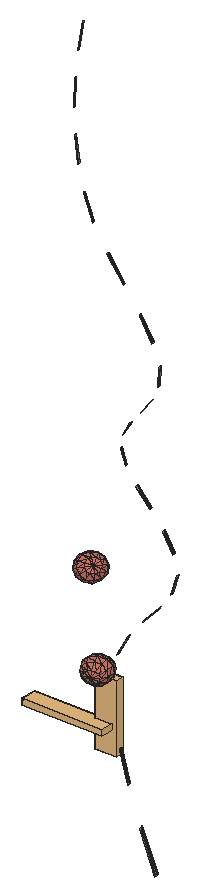
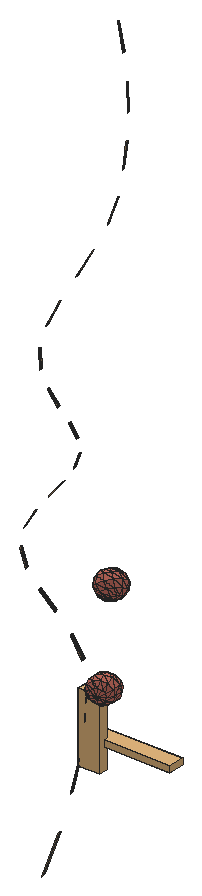
# SketchUp Ruby script. Lengths in inches.
U = 1.inch
M = Sketchup.active_model
def pt(a) = Geom::Point3d.new(a.map { |v| v * U })
def face(e, loops, mat)
  f = e.add_face(loops[0].map { |a| pt(a) })
  loops[1..].each { |l| e.add_face(l.map { |a| pt(a) }).erase! }
  f.material = f.back_material = mat if mat
  f
end
# faces: each face lists its corners as indices into pts; further lists are holes
def faces(e, pts, list, mat = nil) = list.each { |f| face(e, (f[0].is_a?(Array) ? f : [f]).map { |l| l.map { |i| pts[i] } }, mat) }
# xy, xz, yz: faces in a plane at the given z, y or x. An outline is a flat list of corners, or four numbers for a rectangle; further outlines are holes
def ring(l) = l.size == 4 ? [[l[0], l[1]], [l[2], l[1]], [l[2], l[3]], [l[0], l[3]]] : l.each_slice(2).to_a
def flat(e, list, mat, &to3) = list.each { |f| face(e, (f[0].is_a?(Array) ? f : [f]).map { |l| ring(l).map { |u, v| to3.(u, v) } }, mat) }
def xy(e, z, list, mat = nil) = flat(e, list, mat) { |x, y| [x, y, z] }
def xz(e, y, list, mat = nil) = flat(e, list, mat) { |x, z| [x, y, z] }
def yz(e, x, list, mat = nil) = flat(e, list, mat) { |y, z| [x, y, z] }
def lines(e, pts, list) = list.each { |a, b| e.add_line(pt(pts[a]), pt(pts[b])) }
# prism: a flat outline (further loops are holes) pulled along v
def prism(e, loops, v, mat = nil)
  f = face(e, loops, mat); d = Geom::Vector3d.new(v.map { |x| x * U })
  f.pushpull(f.normal.samedirection?(d) ? d.length : -d.length)
end
def box(e, o, s, mat = nil) = prism(e, [[o, [o[0] + s[0], o[1], o[2]], [o[0] + s[0], o[1] + s[1], o[2]], [o[0], o[1] + s[1], o[2]]]], [0, 0, s[2]], mat)
def at(x, y, z, deg = 0) = Geom::Transformation.translation(pt([x, y, z])) * Geom::Transformation.rotation(ORIGIN, Z_AXIS, deg.degrees)
def axes(o, x, y, z) = Geom::Transformation.new([*x, 0, *y, 0, *z, 0, *pt(o).to_a, 1])
def part(name) = M.definitions.add(name)
# library, detail: a bought-in or finely detailed component or shape, given as its bounding box
def library(name, o, s) = part(name).tap { |d| box(d.entities, o, s) }
def detail(e, o, s) = box(e.add_group.entities, o, s)
def put(e, d, t, mat = nil) = e.add_instance(d, t).tap { |i| i.material = mat if mat }
def group(e, t, mat = nil) = e.add_group.tap { |g| g.transformation = t; g.material = mat if mat }.entities
root = M.entities
M.materials.add("green").color = [174, 139, 102]
M.materials.add("vio").color = [206, 114, 100]
c1 = library("3DGeom~98_Defintion",[-97.72,-35.49,-500],[195.44,70.98,1000])
c2 = part("3DGeom~99_Defintion")
p = [[97.72,22.79,-497.94],[82.82,12.47,-499.74],[76.21,14.6,-500],[97.72,22.79,-497.94],[76.21,14.6,-500],[71.74,19.25,-499.92],
  [97.72,22.79,-497.94],[71.74,19.25,-499.92],[70.59,25.16,-499.53],[97.72,22.79,-497.94],[89.78,13.42,-499.21],[82.82,12.47,-499.74],
  [97.72,22.79,-497.94],[70.59,25.16,-499.53],[73.07,30.76,-498.92],[97.72,22.79,-497.94],[95.24,17.19,-498.55],[89.78,13.42,-499.21],
  [97.72,22.79,-497.94],[73.07,30.76,-498.92],[78.53,34.54,-498.26],[97.72,22.79,-497.94],[78.53,34.54,-498.26],[85.49,35.49,-497.73],
  [97.72,22.79,-497.94],[85.49,35.49,-497.73],[92.1,33.35,-497.47],[97.72,22.79,-497.94],[92.1,33.35,-497.47],[96.57,28.7,-497.55],
  [-93.36,-33.24,487.31],[-75.65,-25.4,500],[-97.72,-22.56,484.25],[-93.36,-33.24,487.31],[-97.72,-22.56,484.25],[-96.91,-28.5,484.8],
  [-97.72,-22.56,484.25],[-75.65,-25.4,500],[-91.05,-13.3,489.05],[-97.72,-22.56,484.25],[-91.05,-13.3,489.05],[-95.58,-16.99,485.8],
  [-82.33,-34.66,495.19],[-93.36,-33.24,487.31],[-88.02,-35.49,491.12],[-82.33,-34.66,495.19],[-75.65,-25.4,500],[-93.36,-33.24,487.31],
  [-91.05,-13.3,489.05],[-75.65,-25.4,500],[-80.01,-14.72,496.93],[-91.05,-13.3,489.05],[-80.01,-14.72,496.93],[-85.35,-12.47,493.125],
  [-75.65,-25.4,500],[-82.33,-34.66,495.19],[-77.8,-30.96,498.44],[-75.65,-25.4,500],[-76.46,-19.45,499.45],[-80.01,-14.72,496.93]]
faces(c2.entities,p,[[0,1,2],[3,4,5],[6,7,8],[9,10,11],[12,13,14],[15,16,17],[18,19,20],[21,22,23],
  [24,25,26],[27,28,29],[30,31,32],[33,34,35],[36,37,38],[39,40,41],[42,43,44],[45,46,47],
  [48,49,50],[51,52,53],[54,55,56],[57,58,59]],"green")
c3 = part("3DGeom~243_Defintion")
p = [[-200.91,-81.6,-448.49],[84.65,14.19,-493.26],[-94.16,-142.9,-462.11],[213.68,-130.85,-425.83],[389.77,0,-314.38],[-100.26,120.37,-469.67],
  [240.77,167.48,-392.24],[389.77,0,-314.38],[-311.32,-59.16,-385.97],[-291.49,159.24,-361.38],[27.26,290.09,-365],[-19.66,-226.64,-423.18],
  [-247.73,-261.7,-307.14],[-247.73,-261.7,-307.14],[-247.73,-261.7,-307.14],[252.27,-275.9,-285.45],[213.68,-130.85,-425.83],[434.32,-167.48,-152.28],
  [252.27,-275.9,-285.45],[213.68,-130.85,-425.83],[389.77,0,-314.38],[2.62,-310.38,-342.13],[-247.73,-261.7,-307.14],[252.27,-275.9,-285.45],
  [2.62,-310.38,-342.13],[240.77,167.48,-392.24],[461.41,130.85,-118.6875],[240.77,167.48,-392.24],[332.38,275.9,-186.12],[332.38,275.9,-186.12],
  [-395.79,-81.6,-291.3],[-247.73,-261.7,-307.14],[-395.79,-81.6,-291.3],[-291.49,159.24,-361.38],[-311.32,-59.16,-385.97],[-193.55,334.96,-239.96],
  [147.48,382.07,-162.53],[332.38,275.9,-186.12],[-193.55,334.96,-239.96],[147.48,382.07,-162.53],[27.26,290.09,-365],[-395.79,-81.6,-291.3],
  [-437.8,120.37,-197.41],[-291.49,159.24,-361.38],[-193.55,334.96,-239.96],[-291.49,159.24,-361.38],[2.62,-310.38,-342.13],[190.07,-382.08,-109.73],
  [-33.29,-371.6875,-240.68],[252.27,-275.9,-285.45],[-247.73,-261.7,-307.14],[500,-14.19,21.69],[-117.77,-394.125,-146.01],[-228.17,-371.6875,-83.49],
  [-334.93,-310.38,-69.87],[-334.93,-310.38,-69.87],[-409.43,-226.64,-108.8],[-247.73,-261.7,-307.14],[-431.7,-142.9,-189.85],[-395.79,-81.6,-291.3],
  [-247.73,-261.7,-307.14],[-247.73,-261.7,-307.14],[-395.79,-81.6,-291.3],[252.27,-275.9,-285.45],[362.5,-290.09,50.625],[190.07,-382.08,-109.73],
  [252.27,-275.9,-285.45],[362.5,-290.09,50.625],[43.75,-420.9375,54.25],[-362.5,290.09,-50.625],[-193.55,334.96,-239.96],[-362.5,290.09,-50.625],
  [-43.75,420.9375,-54.25],[-193.55,334.96,-239.96],[-193.55,334.96,-239.96],[147.48,382.07,-162.53],[-500,14.19,-21.69],[409.43,226.64,108.8],
  [334.93,310.39,69.87],[147.48,382.07,-162.53],[334.93,310.39,69.87],[332.38,275.9,-186.12],[147.48,382.07,-162.53],[228.17,371.6875,83.49],
  [334.93,310.39,69.87],[147.48,382.07,-162.53],[437.8,-120.37,197.41],[362.5,-290.09,50.625],[-147.48,-382.08,162.53],[431.7,142.9,189.85],
  [193.55,-334.97,239.96],[362.5,-290.09,50.625],[-461.41,-130.85,118.6875],[-332.38,-275.9,186.12],[-332.38,-275.9,186.12],[-334.93,-310.38,-69.87],
  [-332.38,-275.9,186.12],[-362.5,290.09,-50.625],[-190.07,382.08,109.73],[117.77,394.125,146.01],[-434.32,167.48,152.28],[-190.07,382.08,109.73],
  [395.79,81.6,291.3],[362.5,-290.09,50.625],[291.49,-159.24,361.38],[193.55,-334.97,239.96],[362.5,-290.09,50.625],[-27.26,-290.09,365],
  [-27.26,-290.09,365],[247.73,261.7,307.14],[334.93,310.39,69.87],[247.73,261.7,307.14],[247.73,261.7,307.14],[247.73,261.7,307.14],
  [-252.27,275.9,285.45],[-190.07,382.08,109.73],[-252.27,275.9,285.45],[33.29,371.6875,240.68],[-389.77,0,314.38],[247.73,261.7,307.14],
  [-147.48,-382.08,162.53],[-240.77,-167.48,392.24],[-332.38,-275.9,186.12],[-147.48,-382.08,162.53],[-27.26,-290.09,365],[-240.77,-167.48,392.24],
  [-240.77,-167.48,392.24],[247.73,261.7,307.14],[311.32,59.16,385.97],[193.55,-334.97,239.96],[100.26,-120.37,469.67],[193.55,-334.97,239.96],
  [291.49,-159.24,361.38],[-2.62,310.39,342.13],[247.73,261.7,307.14],[-252.27,275.9,285.45],[-213.68,130.85,425.83],[-213.68,130.85,425.83],
  [-2.62,310.39,342.13],[-252.27,275.9,285.45],[311.32,59.16,385.97],[395.79,81.6,291.3],[247.73,261.7,307.14],[200.91,81.6,448.49],
  [311.32,59.16,385.97],[94.16,142.9,462.11],[19.66,226.64,423.18],[-2.62,310.39,342.13],[-240.77,-167.48,392.24],[-213.68,130.85,425.83],
  [-389.77,0,314.38],[-213.68,130.85,425.83],[-2.62,310.39,342.13],[291.49,-159.24,361.38],[291.49,-159.24,361.38],[311.32,59.16,385.97],
  [-84.65,-14.19,493.26],[-240.77,-167.48,392.24],[-240.77,-167.48,392.24],[-213.68,130.85,425.83],[-213.68,130.85,425.83]]
faces(c3.entities,p,[[0,1,2],[2,1,3],[1,4,3],[0,5,1],[1,6,7],[5,6,1],[8,5,0],[8,9,5],
  [9,10,5],[5,10,6],[2,11,12],[0,2,13],[2,3,11],[8,0,14],[11,3,15],[16,17,18],
  [19,20,17],[11,21,22],[11,23,24],[25,26,20],[27,28,26],[10,29,6],[30,8,31],[32,33,34],
  [9,35,10],[10,36,37],[38,39,40],[41,42,43],[42,44,45],[46,47,48],[46,49,47],[46,48,50],
  [20,51,17],[20,26,51],[48,52,50],[52,53,50],[53,54,50],[55,56,57],[58,59,60],[56,58,61],
  [58,42,62],[63,64,65],[66,17,67],[48,68,52],[48,47,68],[42,69,70],[71,72,73],[74,72,75],
  [58,76,42],[76,69,42],[56,76,58],[28,77,26],[28,78,77],[79,80,81],[82,83,84],[72,83,85],
  [17,86,87],[17,51,86],[52,68,88],[52,88,53],[26,89,51],[26,77,89],[47,90,68],[47,91,90],
  [55,92,56],[56,92,76],[53,88,93],[53,94,95],[55,96,92],[97,98,72],[72,99,83],[98,99,72],
  [76,100,69],[100,101,69],[92,100,76],[51,102,86],[51,89,102],[103,104,105],[106,86,104],[68,107,88],
  [68,90,108],[77,78,109],[110,83,111],[83,99,112],[89,77,113],[100,114,115],[116,117,98],[98,117,99],
  [96,118,92],[92,118,100],[99,117,119],[118,114,100],[120,121,122],[123,124,125],[96,126,118],[102,89,127],
  [86,128,104],[86,102,128],[129,130,124],[131,132,130],[117,133,134],[135,133,117],[118,136,114],[137,138,139],
  [140,141,142],[143,144,142],[145,143,142],[146,145,142],[147,146,142],[148,149,150],[151,146,152],[153,143,130],
  [154,155,143],[124,156,157],[124,130,156],[158,156,159],[156,146,160],[156,145,146],[130,143,145],[130,145,156]],"vio")
c4 = part("3DGeom~210_Defintion")
p = [[-113.26,0,-500],[131.5625,-217.6,-424.04],[-130.88,-188.44,-443.1875],[151.92,0,-489.64],[-348.08,0,-376.38],[-358.26,108.8,-343.58],
  [-130.88,188.44,-443.1875],[-358.26,108.8,-343.58],[-348.08,0,-376.38],[358.76,-188.44,-291.27],[376.38,0,-348.08],[358.76,-188.44,-291.27],
  [131.5625,217.6,-424.04],[75.96,-376.89,-244.82],[-179.04,-326.4,-287.98],[75.96,-376.89,-244.82],[-358.26,-108.8,-343.58],[-179.04,-326.4,-287.98],
  [-348.08,0,-376.38],[-358.26,-108.8,-343.58],[-386.0625,188.44,-253.97],[-358.26,108.8,-343.58],[-386.0625,188.44,-253.97],[-179.04,326.4,-287.98],
  [131.5625,-217.6,-424.04],[310.6,-326.4,-136.0625],[75.96,-376.89,-244.82],[131.5625,-217.6,-424.04],[358.76,-188.44,-291.27],[358.76,188.44,-291.27],
  [75.96,376.89,-244.82],[358.76,188.44,-291.27],[131.5625,217.6,-424.04],[75.96,376.89,-244.82],[-348.08,0,-376.38],[-358.26,-108.8,-343.58],
  [-489.64,0,-151.92],[-358.26,108.8,-343.58],[376.38,0,-348.08],[489.82,-108.8,-80.46],[358.76,-188.44,-291.27],[376.38,0,-348.08],
  [500,0,-113.26],[358.76,188.44,-291.27],[376.38,0,-348.08],[-358.26,-108.8,-343.58],[-179.04,-326.4,-287.98],[-386.0625,-188.44,-253.97],
  [-386.0625,-188.44,-253.97],[-386.0625,188.44,-253.97],[358.76,-188.44,-291.27],[462.02,-188.44,9.15],[310.6,-326.4,-136.0625],[358.76,-188.44,-291.27],
  [358.76,188.44,-291.27],[489.82,108.8,-80.46],[310.6,326.4,-136.0625],[358.76,188.44,-291.27],[75.96,376.89,-244.82],[310.6,326.4,-136.0625],
  [358.76,188.44,-291.27],[-179.04,-326.4,-287.98],[0,-435.19,0],[-244.82,-376.89,-75.96],[-179.04,-326.4,-287.98],[-179.04,-326.4,-287.98],
  [-244.82,-376.89,-75.96],[-424.04,217.6,-131.5625],[-179.04,326.4,-287.98],[-244.82,376.89,-75.96],[-179.04,326.4,-287.98],[-244.82,376.89,-75.96],
  [75.96,376.89,-244.82],[-179.04,326.4,-287.98],[-424.04,-217.6,-131.5625],[244.82,-376.89,75.96],[0,435.19,0],[75.96,376.89,-244.82],
  [-244.82,376.89,-75.96],[75.96,376.89,-244.82],[-462.02,-188.44,-9.15],[-489.82,-108.8,80.46],[-500,0,113.26],[-489.82,108.8,80.46],
  [-462.02,188.44,-9.15],[310.6,-326.4,-136.0625],[424.04,-217.6,131.5625],[244.82,-376.89,75.96],[310.6,-326.4,-136.0625],[310.6,326.4,-136.0625],
  [462.02,188.44,9.15],[244.82,376.89,75.96],[310.6,326.4,-136.0625],[244.82,376.89,75.96],[-310.6,-326.4,136.0625],[489.64,0,151.92],
  [-244.82,-376.89,-75.96],[-75.96,-376.89,244.82],[-244.82,-376.89,-75.96],[-310.6,-326.4,136.0625],[-310.6,326.4,136.0625],[-310.6,326.4,136.0625],
  [-244.82,376.89,-75.96],[-358.76,-188.44,291.27],[179.04,-326.39,287.98],[179.04,-326.39,287.98],[-310.6,326.4,136.0625],[-75.96,376.89,244.82],
  [424.04,217.6,131.5625],[244.82,376.89,75.96],[244.82,-376.89,75.96],[386.0625,-188.44,253.97],[179.04,-326.39,287.98],[244.82,-376.89,75.96],
  [386.0625,-188.44,253.97],[179.04,326.4,287.98],[244.82,376.89,75.96],[179.04,326.4,287.98],[-376.38,0,348.08],[-358.76,188.44,291.27],
  [386.0625,-188.44,253.97],[386.0625,188.44,253.97],[179.04,326.4,287.98],[-310.6,-326.4,136.0625],[-131.5625,-217.6,424.04],[-310.6,-326.4,136.0625],
  [-131.5625,-217.6,424.04],[-358.76,-188.44,291.27],[-358.76,188.44,291.27],[-310.6,326.4,136.0625],[358.26,-108.8,343.58],[386.0625,-188.44,253.97],
  [348.08,0,376.38],[358.26,-108.8,343.58],[358.26,108.8,343.58],[348.08,0,376.38],[358.26,108.8,343.58],[-75.96,-376.89,244.82],
  [130.88,-188.44,443.1875],[-131.5625,-217.6,424.04],[-75.96,-376.89,244.82],[179.04,-326.39,287.98],[-358.76,188.44,291.27],[-131.5625,217.6,424.04],
  [-131.5625,217.6,424.04],[179.04,326.4,287.98],[-75.96,376.89,244.82],[386.0625,-188.44,253.97],[358.26,-108.8,343.58],[130.88,188.44,443.1875],
  [358.26,108.8,343.58],[386.0625,188.44,253.97],[386.0625,188.44,253.97],[179.04,326.4,287.98],[-131.5625,217.6,424.04],[179.04,326.4,287.98],
  [-358.76,-188.44,291.27],[-151.92,0,489.64],[-358.76,-188.44,291.27],[-376.38,0,348.08],[-376.38,0,348.08],[-131.5625,217.6,424.04],
  [-358.76,188.44,291.27],[348.08,0,376.38],[113.26,0,500],[-376.38,0,348.08],[-131.5625,217.6,424.04],[-131.5625,217.6,424.04]]
faces(c4.entities,p,[[0,1,2],[0,3,1],[4,0,2],[5,6,0],[7,0,8],[6,3,0],[3,9,1],[3,10,11],
  [6,12,3],[12,10,3],[2,13,14],[2,1,15],[16,2,17],[18,2,19],[20,6,21],[22,23,6],
  [23,12,6],[24,25,26],[27,28,25],[12,29,10],[30,31,32],[23,33,12],[34,35,36],[37,34,36],
  [38,39,40],[41,42,39],[43,42,44],[45,46,47],[35,48,36],[49,37,36],[50,51,52],[53,39,51],
  [54,55,42],[56,55,57],[58,59,60],[61,62,63],[64,26,62],[48,65,66],[67,68,49],[67,69,70],
  [71,72,73],[48,66,74],[48,74,36],[67,49,36],[26,75,62],[26,25,75],[76,59,77],[78,76,79],
  [74,80,36],[80,81,36],[81,82,36],[82,83,36],[83,84,36],[84,67,36],[85,86,87],[88,51,86],
  [89,90,55],[91,90,92],[76,93,59],[74,66,94],[74,94,80],[84,69,67],[39,42,95],[42,55,95],
  [51,39,95],[55,90,95],[96,62,97],[98,97,99],[84,100,69],[101,76,102],[80,94,103],[80,103,81],
  [83,100,84],[62,104,97],[62,75,105],[106,107,76],[107,93,76],[86,51,95],[90,108,95],[109,108,90],
  [110,111,112],[113,86,114],[115,108,116],[107,117,93],[81,103,118],[81,118,82],[82,119,83],[83,119,100],
  [82,118,119],[120,86,95],[108,121,95],[122,121,108],[123,97,124],[125,126,127],[128,107,129],[130,131,95],
  [132,133,95],[134,135,95],[121,136,95],[137,138,139],[140,141,138],[142,143,107],[144,145,146],[141,147,148],
  [149,150,151],[149,152,153],[141,148,138],[154,149,155],[156,139,157],[158,157,159],[160,161,162],[138,148,163],
  [164,163,150],[164,150,149],[165,157,166],[138,163,164],[139,164,157],[139,138,164],[157,149,167],[157,164,149]],"vio")
c5 = library("3DGeom~78_Defintion",[-59.29,-500,-155.55],[118.58,1000,311.1])
c6 = part("3DGeom~79_Defintion")
p = [[38.96,500,-125.75],[48.07,490.68,-155.1],[39.67,491.3,-155.55],[38.96,500,-125.75],[39.67,491.3,-155.55],[32.3,493.01,-151.95],
  [38.96,500,-125.75],[55.25,491.3,-150.72],[48.07,490.68,-155.1],[38.96,500,-125.75],[32.3,493.01,-151.95],[27.93,495.34,-145.26],
  [38.96,500,-125.75],[59.29,493.01,-143.58],[55.25,491.3,-150.72],[38.96,500,-125.75],[27.93,495.34,-145.26],[27.74,497.67,-137.28],
  [38.96,500,-125.75],[59.1,495.34,-135.59],[59.29,493.01,-143.58],[38.96,500,-125.75],[27.74,497.67,-137.28],[31.78,499.375,-130.14],
  [38.96,500,-125.75],[54.74,497.67,-128.9],[59.1,495.34,-135.59],[38.96,500,-125.75],[47.37,499.375,-125.3],[54.74,497.67,-128.9],
  [-35.57,-494.09,114.48],[-51.43,-495.57,117.9],[-44,-494.49,114.1],[-35.57,-494.09,114.48],[-45.02,-500,144.93],[-51.43,-495.57,117.9],
  [-24.4375,-495.57,126.28],[-45.02,-500,144.93],[-35.57,-494.09,114.48],[-24.4375,-495.57,126.28],[-35.57,-494.09,114.48],[-28.41,-494.49,118.9375],
  [-51.43,-495.57,117.9],[-45.02,-500,144.93],[-56.15,-498.52,133.13],[-51.43,-495.57,117.9],[-56.15,-498.52,133.13],[-55.88,-497.04,124.87],
  [-29.16,-498.52,141.51],[-45.02,-500,144.93],[-24.4375,-495.57,126.28],[-29.16,-498.52,141.51],[-24.4375,-495.57,126.28],[-24.71,-497.04,134.54],
  [-45.02,-500,144.93],[-52.18,-499.6,140.47],[-56.15,-498.52,133.13],[-45.02,-500,144.93],[-29.16,-498.52,141.51],[-36.59,-499.6,145.31]]
faces(c6.entities,p,[[0,1,2],[3,4,5],[6,7,8],[9,10,11],[12,13,14],[15,16,17],[18,19,20],[21,22,23],
  [24,25,26],[27,28,29],[30,31,32],[33,34,35],[36,37,38],[39,40,41],[42,43,44],[45,46,47],
  [48,49,50],[51,52,53],[54,55,56],[57,58,59]],"green")
c7 = part("3DGeom~66_Defintion")
p = [[6.02,125.75,-55.09],[9.11,102.59,-61.04],[7.6875,102.5625,-61.3125],[7.47,125.77,-54.82],[7.72,78.45,-56.27],[8.13,55.5,-43.21],
  [6.76,55.43,-43.46],[9.12,78.5,-56.01],[-0.23,167.06,-22.8125],[4.58,146.58,-40.46],[3.1,146.57,-40.73],[1.28,167.07,-22.54],
  [10.48,-111.71,-34],[11.13,-135.59,-35.53],[9.98,-135.56,-35.72],[11.65,-111.73,-33.8],[8.82,470.02,-32.05],[5.8125,417.1,-14.72],
  [4.01,417.15,-15.03],[10.68,469.97,-31.74],[7.29,-163.17,-28.46],[3.95,-193.64,-14.78],[2.875,-193.58,-14.96],[8.4,-163.22,-28.27],
  [5.29,33.31,-26.85],[5.1,12.08,-9.87],[3.78,12.01,-10.11],[6.64,33.37,-26.61],[7.26,-74.92,-12.89],[10.52,-91.91,-24.9],
  [9.33,-91.9,-25.11],[8.47,-74.92,-12.68],[-5.35,214.57,8.06],[-1.73,189.15,-5.04],[-3.27,189.15,-5.31],[-3.78,214.56,8.32],
  [0.14,368.22,-1.9375],[-1.09,323.22,7.52],[-2.78,323.25,7.23],[1.89,368.18,-1.64],[3.16,-43.84,7.38],[6.22,-59.32,-0.74],
  [4.99,-59.33,-0.96],[4.41,-43.82,7.62],[-2.43,-226.0625,1.91],[-6.8,-259.76,19.51],[-7.8,-259.72,19.34],[-1.39,-226.12,2.09],
  [2.65,-8.27,3.13],[3.59,-27.07,9.68],[2.32,-27.1,9.44],[3.94,-8.22,3.375],[-4.77,282.25,12.47],[-4.22,245.22,14.07],
  [-5.82,245.24,13.8],[-3.125,282.22,12.75],[-12.4375,-293.59,34.51],[-14.57,-326.7,44.78],[-15.51,-326.68,44.63],[-11.46,-293.625,34.67],
  [-16.76,-495.13,51.04],[-14.12,-529.96,45.86],[-14.84,-529.98,45.75],[-16,-495.12,51.16],[-17.21,-359.6,50.29],[-17.3125,-392.91,53.9],
  [-18.18,-392.91,53.76],[-16.3,-359.61,50.43],[-18.43,-426.6,55.04],[-17.16,-460.67,54.26],[-17.96,-460.68,54.13],[-17.6,-426.6,55.17]]
faces(c7.entities,p,[[0,1,2],[0,3,1],[4,5,6],[4,7,5],[8,9,10],[8,11,9],[12,13,14],[12,15,13],
  [16,17,18],[16,19,17],[20,21,22],[20,23,21],[24,25,26],[24,27,25],[28,29,30],[28,31,29],
  [32,33,34],[32,35,33],[36,37,38],[36,39,37],[40,41,42],[40,43,41],[44,45,46],[44,47,45],
  [48,49,50],[48,51,49],[52,53,54],[52,55,53],[56,57,58],[56,59,57],[60,61,62],[60,63,61],
  [64,65,66],[64,67,65],[68,69,70],[68,71,69]],"green")
c8 = part("3DGeom~70_Defintion")
p = [[4.6,125.58,-54.99],[6.02,125.73,-55.08],[7.6875,102.54,-61.3],[6.29,102.51,-61.18],[7.47,125.74,-54.81],[10.41,102.59,-60.39],
  [9.11,102.57,-61.03],[8.81,125.62,-54.19],[6.35,78.48,-56.16],[7.72,78.43,-56.26],[6.76,55.42,-43.45],[5.41,55.51,-43.38],
  [9.12,78.48,-56],[9.39,55.7,-42.65],[8.13,55.48,-43.2],[10.4,78.64,-55.4],[-1.7,166.83,-22.75],[3.1,146.54,-40.72],
  [1.67,146.34,-40.66],[-0.23,167.03,-22.81],[1.28,167.03,-22.54],[5.96,146.36,-39.87],[4.58,146.55,-40.45],[2.68,166.82,-21.96],
  [5.96,146.36,-39.87],[9.33,-111.73,-33.88],[9.98,-135.53,-35.71],[8.86,-135.47,-35.6],[10.48,-111.6875,-33.99],[11.65,-111.71,-33.79],
  [12.19,-135.57,-35.03],[11.13,-135.5625,-35.52],[12.73,-111.79,-33.3],[7.02,470.09,-31.89],[8.82,469.93,-32.05],[4.01,417.0625,-15.03],
  [2.26,417.2,-14.87],[10.67,469.875,-31.73],[7.47,417.07,-13.96],[5.8125,417.02,-14.72],[12.38,469.95,-30.95],[6.2,-163.01,-28.36],
  [7.28,-163.14,-28.46],[2.87,-193.54,-14.96],[1.83,-193.4,-14.88],[8.4,-163.1875,-28.26],[4.95,-193.56,-14.33],[3.95,-193.6,-14.77],
  [9.43,-163.16,-27.8],[3.97,33.4,-26.78],[3.77,12.01,-10.1],[2.48,12.11,-10.04],[5.29,33.3,-26.84],[6.64,33.37,-26.6],
  [6.31,12.3,-9.34],[5.1,12.08,-9.87],[7.88,33.6,-26.08],[6.31,12.3,-9.34],[6.08,-75.06,-12.84],[9.32,-91.88,-25.1],
  [8.16,-92,-25.02],[7.26,-74.91,-12.89],[8.47,-74.91,-12.67],[11.62,-92.03,-24.42],[10.52,-91.89,-24.9],[9.59,-75.0625,-12.2],
  [-6.88,214.4375,8.1875],[-3.27,189.12,-5.31],[-4.77,188.95,-5.22],[-5.35,214.53,8.05],[-3.78,214.51,8.32],[-0.3125,188.92,-4.43],
  [-1.73,189.11,-5.04],[-2.34,214.39,8.98],[-1.56,368.26,-1.78],[0.14,368.15,-1.9375],[-2.78,323.18,7.23],[-4.44,323.27,7.38],
  [1.89,368.1,-1.64],[0.48,323.17,8.24],[-1.09,323.15,7.51],[3.51,368.15,-0.9],[1.9375,-43.9375,7.47],[4.99,-59.32,-0.96],
  [3.79,-59.47,-0.91],[3.16,-43.83,7.38],[4.41,-43.82,7.62],[7.36,-59.44,-0.24],[6.22,-59.31,-0.74],[5.56,-43.88,8.17],
  [-3.44,-225.87,1.98],[-2.43,-226.02,1.91],[-7.8,-259.66,19.34],[-8.78,-259.53,19.41],[-1.39,-226.07,2.09],[-5.86,-259.67,19.92],
  [-6.8,-259.71,19.51],[-0.42,-226.02,2.52],[1.375,-8.2,3.21],[2.65,-8.27,3.13],[2.32,-27.1,9.4375],[1.07,-27.1,9.54],
  [3.94,-8.21,3.375],[4.75,-27.02,10.26],[3.59,-27.07,9.68],[5.13,-8.04,3.92],[-6.38,282.24,12.63],[-4.77,282.19,12.47],
  [-5.82,245.1875,13.79],[-7.38,245.2,13.95],[-3.125,282.16,12.75],[-2.76,245.14,14.75],[-4.22,245.17,14.07],[-1.61,282.16,13.46],
  [-13.375,-293.42,34.59],[-12.43,-293.53,34.5],[-15.51,-326.61,44.62],[-16.42,-326.55,44.71],[-11.46,-293.57,34.67],[-13.71,-326.61,45.16],
  [-14.57,-326.63,44.77],[-10.5625,-293.53,35.07],[-17.5,-495.0625,51.1],[-16.76,-495.03,51.03],[-14.84,-529.87,45.74],[-15.54,-529.91,45.81],
  [-16,-495.02,51.15],[-13.45,-529.86,46.16],[-14.12,-529.85,45.85],[-15.3,-495.03,51.46],[-18.08,-359.49,50.37],[-17.2,-359.53,50.28],
  [-18.18,-392.83,53.75],[-19.02,-392.8125,53.84],[-16.3,-359.54,50.42],[-16.51,-392.83,54.25],[-17.31,-392.83,53.89],[-15.47,-359.53,50.8],
  [-19.23,-426.52,55.12],[-18.43,-426.51,55.03],[-17.95,-460.58,54.125],[-18.73,-460.6,54.21],[-17.6,-426.51,55.16],[-16.43,-460.58,54.58],
  [-17.16,-460.57,54.25],[-16.83,-426.51,55.51]]
faces(c8.entities,p,[[0,1,2],[0,2,3],[4,5,6],[4,7,5],[8,9,10],[8,10,11],[12,13,14],[12,15,13],
  [16,17,18],[16,19,17],[20,21,22],[20,23,24],[25,26,27],[25,28,26],[29,30,31],[29,32,30],
  [33,34,35],[33,35,36],[37,38,39],[37,40,38],[41,42,43],[41,43,44],[45,46,47],[45,48,46],
  [49,50,51],[49,52,50],[53,54,55],[53,56,57],[58,59,60],[58,61,59],[62,63,64],[62,65,63],
  [66,67,68],[66,69,67],[70,71,72],[70,73,71],[74,75,76],[74,76,77],[78,79,80],[78,81,79],
  [82,83,84],[82,85,83],[86,87,88],[86,89,87],[90,91,92],[90,92,93],[94,95,96],[94,97,95],
  [98,99,100],[98,100,101],[102,103,104],[102,105,103],[106,107,108],[106,108,109],[110,111,112],[110,113,111],
  [114,115,116],[114,116,117],[118,119,120],[118,121,119],[122,123,124],[122,124,125],[126,127,128],[126,129,127],
  [130,131,132],[130,132,133],[134,135,136],[134,137,135],[138,139,140],[138,140,141],[142,143,144],[142,145,143]],"green")
g1 = group(root,at(15.3125,134.49,26.21))
put(g1,c1,axes([-1.92,-0.18,7.2],[0,0.00108,0],[0,0,-0.00108],[-0.00108,0,0]),"green")
put(g1,c2,axes([-1.92,-0.18,7.2],[0,0.00108,0],[0,0,-0.00108],[-0.00108,0,0]),"green")
g2 = group(root,at(15.3125,134.49,26.21))
put(g2,c3,axes([-1.65,-0.14,9.04],[0,0.00039,0],[0,0,-0.00039],[-0.00039,0,0]),"vio")
g3 = group(root,at(15.3125,134.49,26.21))
put(g3,c4,axes([-1.58,-0.11,7.8125],[0,0.00038,0],[0,0,-0.00038],[-0.00038,0,0]),"vio")
g4 = group(root,at(15.3125,134.49,26.21))
put(g4,c5,axes([-1.46,-0.07,7.32],[0,0.00091,0],[0,0,-0.00091],[-0.00091,0,0]),"green")
put(g4,c6,axes([-1.46,-0.07,7.32],[0,0.00091,0],[0,0,-0.00091],[-0.00091,0,0]),"green")
put(root,c7,axes([14.0625,134.46,36.46],[0,0.01013,0],[0,0,-0.01013],[-0.01013,0,0]),"green")
put(root,c8,axes([14.0625,134.46,36.46],[0,0.01013,0],[0,0,-0.01013],[-0.01013,0,0]),"green")
